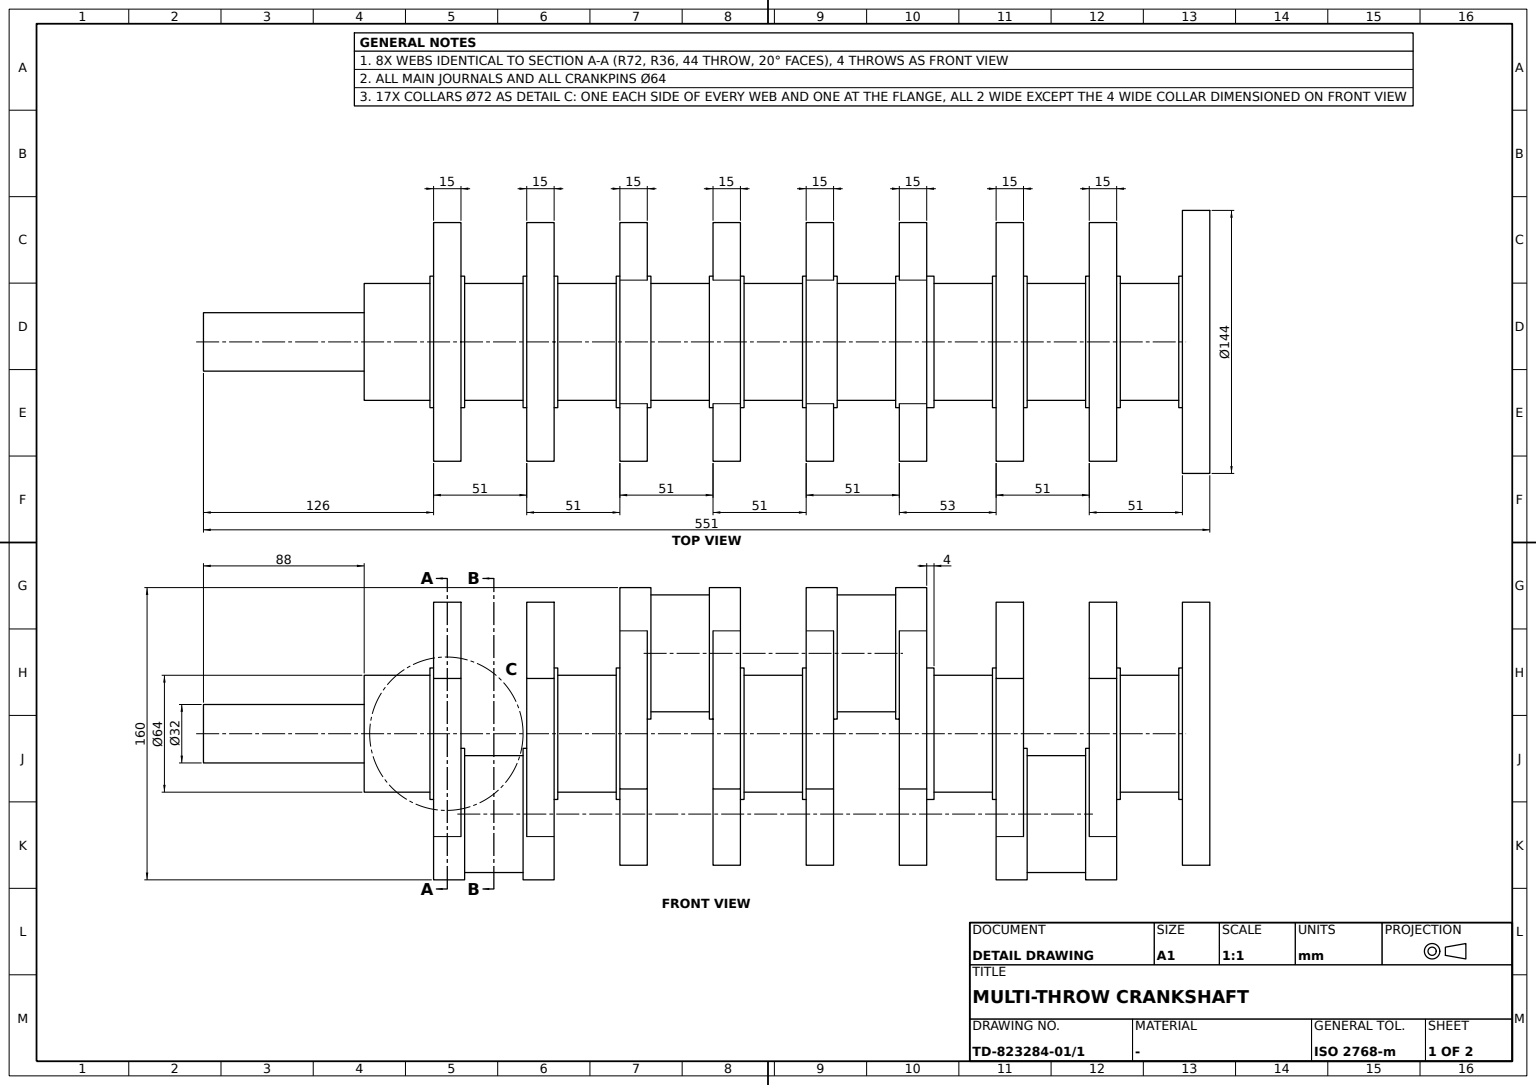
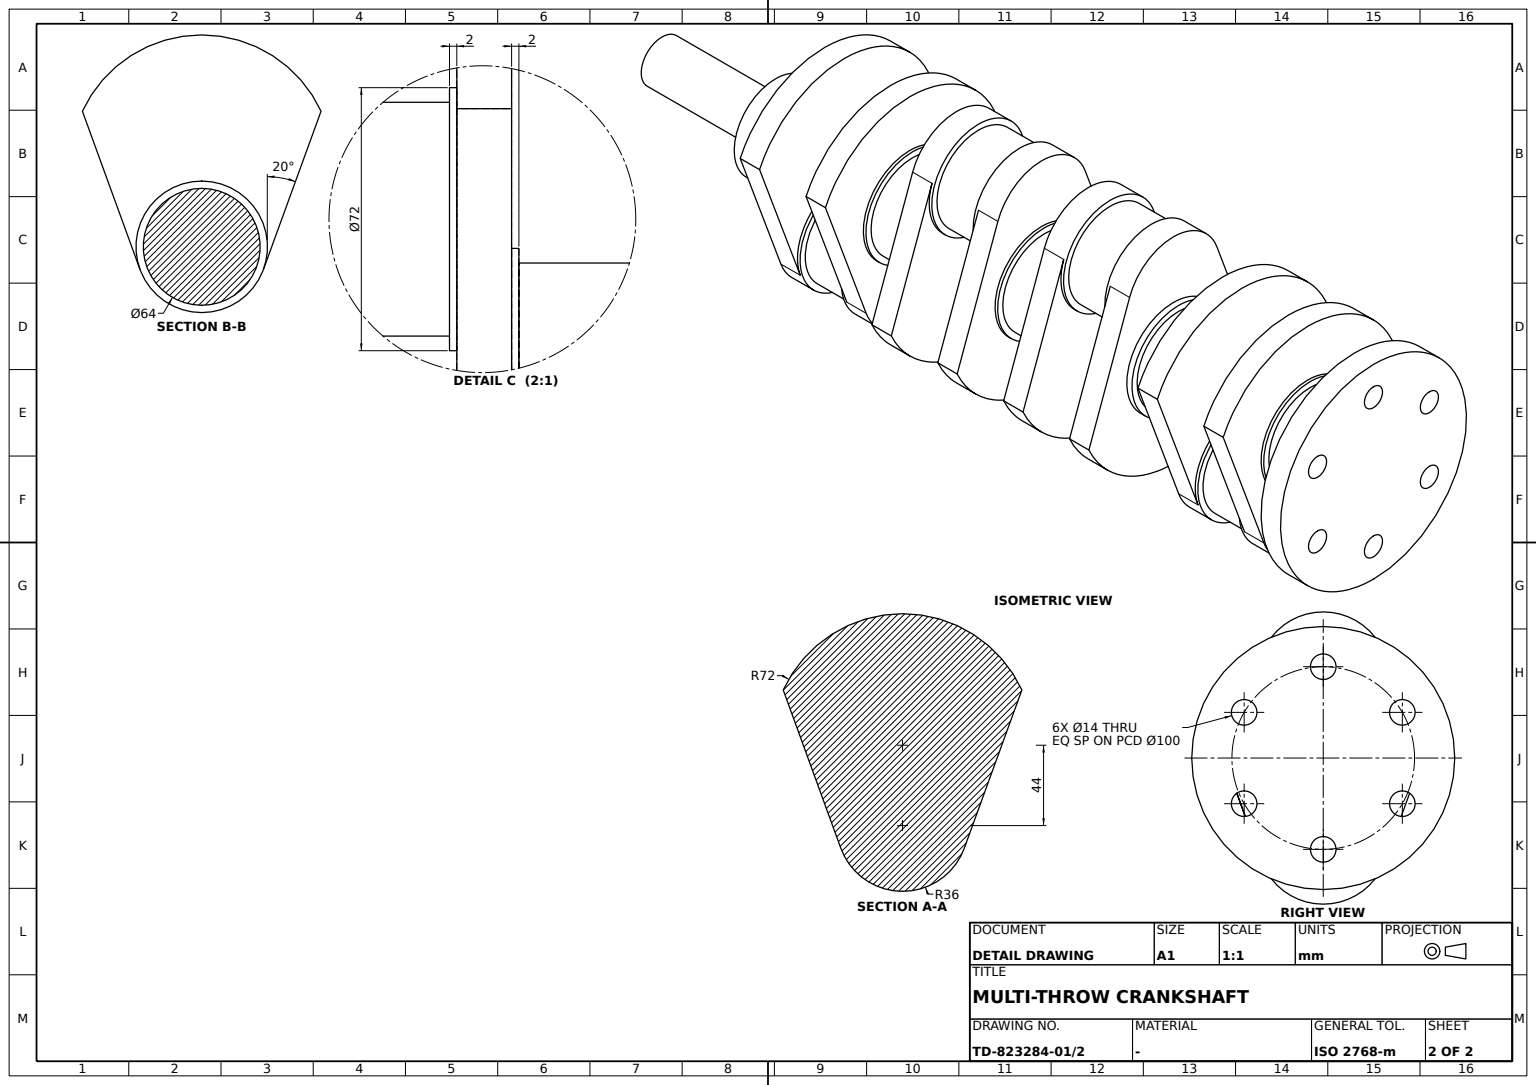
solid
v1 (502,0,-32)
v2 (502,0,32)
e1 v1 v2 CIRCLE(AX(P(502,0,0),D(1,0,0),D(0,1,0)),32)
e2 v2 v1 CIRCLE(AX(P(502,0,0),D(1,0,0),D(0,1,0)),32)
v3 (502,0,-36)
v4 (502,0,36)
e3 v3 v4 CIRCLE(AX(P(502,0,0),D(1,0,0),D(0,1,0)),36)
e4 v4 v3 CIRCLE(AX(P(502,0,0),D(1,0,0),D(0,1,0)),36)
face PLANE(AX(P(502,0,0),D(1,0,0),D(0,0,-1))) [-e1 -e2] [e3 e4]
v5 (296,0,-36)
v6 (296,0,36)
e5 v5 v6 CIRCLE(AX(P(296,0,0),D(1,0,0),D(0,1,0)),36)
v7 (294,0,-36)
e6 v7 v5 LINE
v8 (294,0,36)
e7 v7 v8 CIRCLE(AX(P(294,0,0),D(1,0,0),D(0,1,0)),36)
e8 v6 v8 LINE
face CYL(AX(P(296,0,0),D(-1,0,0),D(0,0,1)),36) [-e5 -e6 e7 -e8]
v9 (500,0,-36)
e9 v9 v3 LINE
v10 (500,0,36)
e10 v9 v10 CIRCLE(AX(P(500,0,0),D(1,0,0),D(0,1,0)),36)
e11 v4 v10 LINE
face CYL(AX(P(502,0,0),D(-1,0,0),D(0,0,1)),36) [-e3 -e9 e10 -e11]
v11 (143,0,-76)
v12 (143,0,-12)
e12 v11 v12 CIRCLE(AX(P(143,0,-44),D(1,0,0),D(0,1,0)),32)
v13 (175,0,-12)
e13 v13 v12 LINE
v14 (175,0,-76)
e14 v14 v13 CIRCLE(AX(P(175,0,-44),D(1,0,0),D(0,1,0)),32)
e15 v11 v14 LINE
face CYL(AX(P(175,0,-44),D(-1,0,0),D(0,0,1)),32) [e12 -e13 -e14 -e15]
v15 (449,65.336033,30.252318)
v16 (434,65.336033,30.252318)
e16 v15 v16 LINE
v17 (449,33.828934,-56.312725)
e17 v17 v15 LINE
v18 (434,33.828934,-56.312725)
e18 v17 v18 LINE
e19 v18 v16 LINE
face PLANE(AX(P(449,33.828934,-56.312725),D(0,-0.939692621,0.342020143),D(0,-0.342020143,-0.939692621))) rev [-e16 -e17 e18 e19]
v19 (396,65.336033,-30.252318)
v20 (396,33.828934,56.312725)
e20 v19 v20 LINE
v21 (381,65.336033,-30.252318)
e21 v19 v21 LINE
v22 (381,33.828934,56.312725)
e22 v21 v22 LINE
e23 v20 v22 LINE
face PLANE(AX(P(396,65.336033,-30.252318),D(0,-0.939692621,-0.342020143),D(0,0.342020143,-0.939692621))) rev [-e20 e21 e22 -e23]
v23 (449,0,72)
v24 (449,-65.336033,30.252318)
e24 v23 v24 CIRCLE(AX(P(449,0,0),D(1,0,0),D(0,0,-1)),72)
v25 (434,0,72)
e25 v23 v25 LINE
v26 (434,-65.336033,30.252318)
e26 v25 v26 CIRCLE(AX(P(434,0,0),D(1,0,0),D(0,0,-1)),72)
e27 v24 v26 LINE
face CYL(AX(P(449,0,0),D(-1,0,0),D(0,0,1)),72) [-e24 e25 e26 -e27]
v27 (294,65.336033,-30.252318)
v28 (294,33.828934,56.312725)
e28 v27 v28 LINE
v29 (294,0,80)
e29 v28 v29 CIRCLE(AX(P(294,0,44),D(1,0,0),D(0,0,-1)),36)
v30 (294,-33.828934,56.312725)
e30 v29 v30 CIRCLE(AX(P(294,0,44),D(1,0,0),D(0,0,-1)),36)
v31 (294,-65.336033,-30.252318)
e31 v30 v31 LINE
e32 v31 v27 CIRCLE(AX(P(294,0,0),D(1,0,0),D(0,0,-1)),72)
e33 v8 v7 CIRCLE(AX(P(294,0,0),D(1,0,0),D(0,1,0)),36)
face PLANE(AX(P(294,0,0),D(1,0,0),D(0,0,-1))) [e28 e29 e30 e31 e32] [-e7 -e33]
v32 (192,-33.828934,-56.312725)
v33 (192,0,-80)
e34 v32 v33 CIRCLE(AX(P(192,0,-44),D(1,0,0),D(0,0,-1)),36)
v34 (177,-33.828934,-56.312725)
e35 v32 v34 LINE
v35 (177,0,-8)
e36 v35 v34 CIRCLE(AX(P(177,0,-44),D(1,0,0),D(0,0,-1)),36)
v36 (175,0,-8)
e37 v35 v36 LINE
v37 (175,0,-80)
e38 v36 v37 CIRCLE(AX(P(175,0,-44),D(1,0,0),D(0,0,-1)),36)
e39 v37 v33 LINE
face CYL(AX(P(177,0,-44),D(-1,0,0),D(0,0,1)),36) [-e34 e35 -e36 e37 e38 e39]
v38 (279,-65.336033,-30.252318)
e40 v31 v38 LINE
v39 (279,-33.828934,56.312725)
e41 v30 v39 LINE
e42 v39 v38 LINE
face PLANE(AX(P(294,-33.828934,56.312725),D(0,0.939692621,-0.342020143),D(0,0.342020143,0.939692621))) rev [-e40 -e31 e41 e42]
v40 (243,0,8)
v41 (245,0,8)
e43 v40 v41 LINE
v42 (245,0,80)
e44 v42 v41 CIRCLE(AX(P(245,0,44),D(1,0,0),D(0,1,0)),36)
v43 (228,0,80)
e45 v42 v43 LINE
v44 (228,-33.828934,56.312725)
e46 v43 v44 CIRCLE(AX(P(228,0,44),D(1,0,0),D(0,1,0)),36)
v45 (243,-33.828934,56.312725)
e47 v45 v44 LINE
e48 v40 v45 CIRCLE(AX(P(243,0,44),D(-1,0,0),D(0,1,0)),36)
face CYL(AX(P(243,0,44),D(-1,0,0),D(0,0,1)),36) [e43 -e44 e45 e46 -e47 -e48]
e49 v37 v36 CIRCLE(AX(P(175,0,-44),D(1,0,0),D(0,0,-1)),36)
v46 (177,33.828934,-56.312725)
e50 v46 v35 CIRCLE(AX(P(177,0,-44),D(1,0,0),D(0,0,-1)),36)
v47 (192,33.828934,-56.312725)
e51 v47 v46 LINE
e52 v33 v47 CIRCLE(AX(P(192,0,-44),D(1,0,0),D(0,0,-1)),36)
face CYL(AX(P(177,0,-44),D(-1,0,0),D(0,0,1)),36) [-e39 e49 -e37 -e50 -e51 -e52]
v48 (141,-33.828934,-56.312725)
v49 (141,0,-8)
e53 v48 v49 CIRCLE(AX(P(141,0,-44),D(-1,0,0),D(0,1,0)),36)
v50 (126,-33.828934,-56.312725)
e54 v48 v50 LINE
v51 (126,0,-80)
e55 v50 v51 CIRCLE(AX(P(126,0,-44),D(1,0,0),D(0,1,0)),36)
v52 (143,0,-80)
e56 v51 v52 LINE
v53 (143,0,-8)
e57 v53 v52 CIRCLE(AX(P(143,0,-44),D(1,0,0),D(0,1,0)),36)
e58 v53 v49 LINE
face CYL(AX(P(141,0,-44),D(-1,0,0),D(0,0,1)),36) [-e53 e54 e55 e56 -e57 e58]
v54 (551,0,72)
v55 (551,0,-72)
e59 v54 v55 CIRCLE(AX(P(551,0,0),D(1,0,0),D(0,1,0)),72)
e60 v55 v54 CIRCLE(AX(P(551,0,0),D(1,0,0),D(0,1,0)),72)
v56 (551,0,43)
v57 (551,0,57)
e61 v56 v57 CIRCLE(AX(P(551,0,50),D(1,0,0),D(0,1,0)),7)
e62 v57 v56 CIRCLE(AX(P(551,0,50),D(1,0,0),D(0,1,0)),7)
v58 (551,0,-57)
v59 (551,0,-43)
e63 v58 v59 CIRCLE(AX(P(551,0,-50),D(1,0,0),D(0,-1,0)),7)
e64 v59 v58 CIRCLE(AX(P(551,0,-50),D(1,0,0),D(0,-1,0)),7)
v60 (551,43.30127,32)
v61 (551,43.30127,18)
e65 v60 v61 CIRCLE(AX(P(551,43.30127,25),D(1,0,0),D(0,0.5,-0.866025404)),7)
e66 v61 v60 CIRCLE(AX(P(551,43.30127,25),D(1,0,0),D(0,0.5,-0.866025404)),7)
v62 (551,-43.30127,-18)
v63 (551,-43.30127,-32)
e67 v62 v63 CIRCLE(AX(P(551,-43.30127,-25),D(1,0,0),D(0,-0.5,0.866025404)),7)
e68 v63 v62 CIRCLE(AX(P(551,-43.30127,-25),D(1,0,0),D(0,-0.5,0.866025404)),7)
v64 (551,43.30127,-32)
v65 (551,43.30127,-18)
e69 v64 v65 CIRCLE(AX(P(551,43.30127,-25),D(1,0,0),D(0,-0.5,-0.866025404)),7)
e70 v65 v64 CIRCLE(AX(P(551,43.30127,-25),D(1,0,0),D(0,-0.5,-0.866025404)),7)
v66 (551,-43.30127,18)
v67 (551,-43.30127,32)
e71 v66 v67 CIRCLE(AX(P(551,-43.30127,25),D(1,0,0),D(0,0.5,0.866025404)),7)
e72 v67 v66 CIRCLE(AX(P(551,-43.30127,25),D(1,0,0),D(0,0.5,0.866025404)),7)
face PLANE(AX(P(551,0,0),D(1,0,0),D(0,0,-1))) [e59 e60] [-e61 -e62] [-e63 -e64] [-e65 -e66] [-e67 -e68] [-e69 -e70] [-e71 -e72]
e73 v13 v14 CIRCLE(AX(P(175,0,-44),D(1,0,0),D(0,1,0)),32)
face PLANE(AX(P(175,0,-44),D(1,0,0),D(0,0,-1))) rev [e14 e73] [-e49 -e38]
v68 (296,0,32)
v69 (328,0,32)
e74 v68 v69 LINE
v70 (328,0,-32)
e75 v70 v69 CIRCLE(AX(P(328,0,0),D(1,0,0),D(0,1,0)),32)
v71 (296,0,-32)
e76 v70 v71 LINE
e77 v71 v68 CIRCLE(AX(P(296,0,0),D(1,0,0),D(0,1,0)),32)
face CYL(AX(P(328,0,0),D(-1,0,0),D(0,0,1)),32) [e74 -e75 e76 e77]
v72 (379,0,8)
v73 (379,0,80)
e78 v72 v73 CIRCLE(AX(P(379,0,44),D(1,0,0),D(0,1,0)),36)
e79 v73 v72 CIRCLE(AX(P(379,0,44),D(1,0,0),D(0,1,0)),36)
v74 (379,0,76)
v75 (379,0,12)
e80 v74 v75 CIRCLE(AX(P(379,0,44),D(1,0,0),D(0,1,0)),32)
e81 v75 v74 CIRCLE(AX(P(379,0,44),D(1,0,0),D(0,1,0)),32)
face PLANE(AX(P(379,0,44),D(1,0,0),D(0,0,-1))) rev [-e78 -e79] [e80 e81]
v76 (141,33.828934,-56.312725)
v77 (141,65.336033,30.252318)
e82 v76 v77 LINE
v78 (126,33.828934,-56.312725)
e83 v76 v78 LINE
v79 (126,65.336033,30.252318)
e84 v78 v79 LINE
e85 v77 v79 LINE
face PLANE(AX(P(141,33.828934,-56.312725),D(0,-0.939692621,0.342020143),D(0,-0.342020143,-0.939692621))) rev [-e82 e83 e84 -e85]
e86 v41 v42 CIRCLE(AX(P(245,0,44),D(1,0,0),D(0,1,0)),36)
v80 (245,0,76)
v81 (245,0,12)
e87 v80 v81 CIRCLE(AX(P(245,0,44),D(1,0,0),D(0,1,0)),32)
e88 v81 v80 CIRCLE(AX(P(245,0,44),D(1,0,0),D(0,1,0)),32)
face PLANE(AX(P(245,0,44),D(1,0,0),D(0,0,-1))) [e86 e44] [-e87 -e88]
v82 (277,0,8)
v83 (279,0,8)
e89 v82 v83 LINE
v84 (277,0,80)
e90 v82 v84 CIRCLE(AX(P(277,0,44),D(1,0,0),D(0,1,0)),36)
e91 v29 v84 LINE
v85 (279,33.828934,56.312725)
e92 v28 v85 LINE
e93 v83 v85 CIRCLE(AX(P(279,0,44),D(1,0,0),D(0,1,0)),36)
face CYL(AX(P(279,0,44),D(-1,0,0),D(0,0,1)),36) [-e89 e90 -e91 -e29 e92 -e93]
v86 (228,-65.336033,-30.252318)
e94 v44 v86 LINE
v87 (243,-65.336033,-30.252318)
e95 v87 v86 LINE
e96 v45 v87 LINE
face PLANE(AX(P(243,-33.828934,56.312725),D(0,0.939692621,-0.342020143),D(0,0.342020143,0.939692621))) rev [e94 -e95 -e96 e47]
v88 (277,0,76)
e97 v80 v88 LINE
v89 (277,0,12)
e98 v89 v88 CIRCLE(AX(P(277,0,44),D(1,0,0),D(0,1,0)),32)
e99 v89 v81 LINE
face CYL(AX(P(277,0,44),D(-1,0,0),D(0,0,1)),32) [e88 e97 -e98 e99]
v90 (347,0,8)
v91 (347,0,80)
e100 v90 v91 CIRCLE(AX(P(347,0,44),D(1,0,0),D(0,1,0)),36)
e101 v91 v90 CIRCLE(AX(P(347,0,44),D(1,0,0),D(0,1,0)),36)
v92 (347,0,76)
v93 (347,0,12)
e102 v92 v93 CIRCLE(AX(P(347,0,44),D(1,0,0),D(0,1,0)),32)
e103 v93 v92 CIRCLE(AX(P(347,0,44),D(1,0,0),D(0,1,0)),32)
face PLANE(AX(P(347,0,44),D(1,0,0),D(0,0,-1))) [e100 e101] [-e102 -e103]
v94 (536,-43.30127,-32)
v95 (536,-43.30127,-18)
e104 v94 v95 CIRCLE(AX(P(536,-43.30127,-25),D(1,0,0),D(0,-0.5,0.866025404)),7)
e105 v94 v63 LINE
e106 v62 v95 LINE
face CYL(AX(P(536,-43.30127,-25),D(1,0,0),D(0,0,-1)),7) rev [-e104 e105 e68 e106]
v96 (432,0,36)
v97 (432,0,-36)
e107 v96 v97 CIRCLE(AX(P(432,0,0),D(1,0,0),D(0,1,0)),36)
e108 v97 v96 CIRCLE(AX(P(432,0,0),D(1,0,0),D(0,1,0)),36)
v98 (432,0,-32)
v99 (432,0,32)
e109 v98 v99 CIRCLE(AX(P(432,0,0),D(1,0,0),D(0,1,0)),32)
e110 v99 v98 CIRCLE(AX(P(432,0,0),D(1,0,0),D(0,1,0)),32)
face PLANE(AX(P(432,0,0),D(1,0,0),D(0,0,-1))) rev [-e107 -e108] [e109 e110]
v100 (328,0,-36)
v101 (330,0,-36)
e111 v100 v101 LINE
v102 (328,0,36)
e112 v100 v102 CIRCLE(AX(P(328,0,0),D(1,0,0),D(0,1,0)),36)
v103 (330,0,36)
e113 v103 v102 LINE
e114 v101 v103 CIRCLE(AX(P(330,0,0),D(1,0,0),D(0,1,0)),36)
face CYL(AX(P(330,0,0),D(-1,0,0),D(0,0,1)),36) [-e111 e112 -e113 -e114]
v104 (194,0,36)
v105 (194,0,-36)
e115 v104 v105 CIRCLE(AX(P(194,0,0),D(1,0,0),D(0,0,-1)),36)
v106 (192,0,36)
e116 v104 v106 LINE
v107 (192,0,-36)
e117 v106 v107 CIRCLE(AX(P(192,0,0),D(1,0,0),D(0,0,-1)),36)
e118 v107 v105 LINE
face CYL(AX(P(194,0,0),D(-1,0,0),D(0,0,1)),36) [-e115 e116 e117 e118]
v108 (536,0,43)
v109 (536,0,57)
e119 v108 v109 CIRCLE(AX(P(536,0,50),D(1,0,0),D(0,1,0)),7)
e120 v109 v108 CIRCLE(AX(P(536,0,50),D(1,0,0),D(0,1,0)),7)
v110 (536,0,72)
v111 (536,0,-72)
e121 v110 v111 CIRCLE(AX(P(536,0,0),D(1,0,0),D(0,1,0)),72)
e122 v111 v110 CIRCLE(AX(P(536,0,0),D(1,0,0),D(0,1,0)),72)
e123 v95 v94 CIRCLE(AX(P(536,-43.30127,-25),D(1,0,0),D(0,-0.5,0.866025404)),7)
v112 (536,43.30127,18)
v113 (536,43.30127,32)
e124 v112 v113 CIRCLE(AX(P(536,43.30127,25),D(1,0,0),D(0,0.5,-0.866025404)),7)
e125 v113 v112 CIRCLE(AX(P(536,43.30127,25),D(1,0,0),D(0,0.5,-0.866025404)),7)
v114 (536,0,-43)
v115 (536,0,-57)
e126 v114 v115 CIRCLE(AX(P(536,0,-50),D(1,0,0),D(0,-1,0)),7)
e127 v115 v114 CIRCLE(AX(P(536,0,-50),D(1,0,0),D(0,-1,0)),7)
v116 (536,0,36)
v117 (536,0,-36)
e128 v116 v117 CIRCLE(AX(P(536,0,0),D(1,0,0),D(0,1,0)),36)
e129 v117 v116 CIRCLE(AX(P(536,0,0),D(1,0,0),D(0,1,0)),36)
v118 (536,-43.30127,18)
v119 (536,-43.30127,32)
e130 v118 v119 CIRCLE(AX(P(536,-43.30127,25),D(1,0,0),D(0,0.5,0.866025404)),7)
e131 v119 v118 CIRCLE(AX(P(536,-43.30127,25),D(1,0,0),D(0,0.5,0.866025404)),7)
v120 (536,43.30127,-18)
v121 (536,43.30127,-32)
e132 v120 v121 CIRCLE(AX(P(536,43.30127,-25),D(1,0,0),D(0,-0.5,-0.866025404)),7)
e133 v121 v120 CIRCLE(AX(P(536,43.30127,-25),D(1,0,0),D(0,-0.5,-0.866025404)),7)
face PLANE(AX(P(536,0,0),D(1,0,0),D(0,0,-1))) rev [e119 e120] [-e121 -e122] [e123 e104] [e124 e125] [e126 e127] [e128 e129] [e130 e131] [e132 e133]
v122 (451,0,-76)
v123 (451,0,-12)
e134 v122 v123 CIRCLE(AX(P(451,0,-44),D(1,0,0),D(0,1,0)),32)
e135 v123 v122 CIRCLE(AX(P(451,0,-44),D(1,0,0),D(0,1,0)),32)
v124 (451,0,-8)
v125 (451,0,-80)
e136 v124 v125 CIRCLE(AX(P(451,0,-44),D(1,0,0),D(0,1,0)),36)
e137 v125 v124 CIRCLE(AX(P(451,0,-44),D(1,0,0),D(0,1,0)),36)
face PLANE(AX(P(451,0,-44),D(1,0,0),D(0,0,-1))) [-e134 -e135] [e136 e137]
v126 (330,0,80)
e138 v126 v91 LINE
v127 (330,-33.828934,56.312725)
e139 v126 v127 CIRCLE(AX(P(330,0,44),D(1,0,0),D(0,0,-1)),36)
v128 (345,-33.828934,56.312725)
e140 v128 v127 LINE
v129 (345,0,8)
e141 v129 v128 CIRCLE(AX(P(345,0,44),D(-1,0,0),D(0,1,0)),36)
e142 v90 v129 LINE
face CYL(AX(P(345,0,44),D(-1,0,0),D(0,0,1)),36) [-e138 e139 -e140 -e141 -e142 -e101]
v130 (124,0,32)
v131 (88,0,32)
e143 v130 v131 LINE
v132 (88,0,-32)
e144 v131 v132 CIRCLE(AX(P(88,0,0),D(1,0,0),D(0,1,0)),32)
v133 (124,0,-32)
e145 v132 v133 LINE
e146 v130 v133 CIRCLE(AX(P(124,0,0),D(1,0,0),D(0,1,0)),32)
face CYL(AX(P(124,0,0),D(-1,0,0),D(0,0,1)),32) [e143 e144 e145 -e146]
v134 (228,33.828934,56.312725)
e147 v134 v43 CIRCLE(AX(P(228,0,44),D(1,0,0),D(0,1,0)),36)
v135 (228,65.336033,-30.252318)
e148 v135 v134 LINE
e149 v86 v135 CIRCLE(AX(P(228,0,0),D(1,0,0),D(0,1,0)),72)
v136 (228,0,36)
v137 (228,0,-36)
e150 v136 v137 CIRCLE(AX(P(228,0,0),D(1,0,0),D(0,0,-1)),36)
e151 v137 v136 CIRCLE(AX(P(228,0,0),D(1,0,0),D(0,0,-1)),36)
face PLANE(AX(P(228,0,0),D(1,0,0),D(0,0,-1))) rev [-e94 -e46 -e147 -e148 -e149] [e150 e151]
v138 (226,0,36)
e152 v136 v138 LINE
v139 (226,0,-36)
e153 v139 v137 LINE
e154 v139 v138 CIRCLE(AX(P(226,0,0),D(1,0,0),D(0,0,-1)),36)
face CYL(AX(P(228,0,0),D(-1,0,0),D(0,0,1)),36) [-e152 -e151 -e153 e154]
v140 (279,65.336033,-30.252318)
e155 v140 v85 LINE
e156 v38 v140 CIRCLE(AX(P(279,0,0),D(1,0,0),D(0,0,-1)),72)
e157 v39 v83 CIRCLE(AX(P(279,0,44),D(1,0,0),D(0,1,0)),36)
face PLANE(AX(P(279,0,0),D(1,0,0),D(0,0,-1))) rev [-e155 -e156 -e42 e157 e93]
v141 (396,-65.336033,-30.252318)
e158 v141 v19 CIRCLE(AX(P(396,0,0),D(1,0,0),D(0,0,-1)),72)
v142 (381,-65.336033,-30.252318)
e159 v141 v142 LINE
e160 v142 v21 CIRCLE(AX(P(381,0,0),D(1,0,0),D(0,0,-1)),72)
face CYL(AX(P(396,0,0),D(-1,0,0),D(0,0,1)),72) [-e21 -e158 e159 e160]
e161 v133 v130 CIRCLE(AX(P(124,0,0),D(1,0,0),D(0,1,0)),32)
e162 v132 v131 CIRCLE(AX(P(88,0,0),D(1,0,0),D(0,1,0)),32)
face CYL(AX(P(124,0,0),D(-1,0,0),D(0,0,1)),32) [-e143 -e161 -e145 e162]
v143 (192,65.336033,30.252318)
v144 (192,0,72)
e163 v143 v144 CIRCLE(AX(P(192,0,0),D(1,0,0),D(0,0,-1)),72)
v145 (177,65.336033,30.252318)
e164 v143 v145 LINE
v146 (177,0,72)
e165 v145 v146 CIRCLE(AX(P(177,0,0),D(1,0,0),D(0,0,-1)),72)
e166 v144 v146 LINE
face CYL(AX(P(192,0,0),D(-1,0,0),D(0,0,1)),72) [-e163 e164 e165 -e166]
v147 (483,0,-76)
v148 (483,0,-12)
e167 v147 v148 CIRCLE(AX(P(483,0,-44),D(1,0,0),D(0,1,0)),32)
e168 v147 v122 LINE
e169 v123 v148 LINE
face CYL(AX(P(483,0,-44),D(-1,0,0),D(0,0,1)),32) [-e167 e168 e134 e169]
e170 v110 v54 LINE
e171 v55 v111 LINE
face CYL(AX(P(551,0,0),D(-1,0,0),D(0,0,1)),72) [e122 e170 -e60 e171]
v149 (500,65.336033,30.252318)
v150 (500,0,72)
e172 v149 v150 CIRCLE(AX(P(500,0,0),D(1,0,0),D(0,0,-1)),72)
v151 (485,65.336033,30.252318)
e173 v149 v151 LINE
v152 (485,0,72)
e174 v151 v152 CIRCLE(AX(P(485,0,0),D(1,0,0),D(0,0,-1)),72)
e175 v150 v152 LINE
face CYL(AX(P(500,0,0),D(-1,0,0),D(0,0,1)),72) [-e172 e173 e174 -e175]
e176 v16 v25 CIRCLE(AX(P(434,0,0),D(1,0,0),D(0,0,-1)),72)
e177 v15 v23 CIRCLE(AX(P(449,0,0),D(1,0,0),D(0,0,-1)),72)
face CYL(AX(P(449,0,0),D(-1,0,0),D(0,0,1)),72) [e176 -e25 -e177 e16]
v153 (485,33.828934,-56.312725)
v154 (485,0,-8)
e178 v153 v154 CIRCLE(AX(P(485,0,-44),D(1,0,0),D(0,1,0)),36)
v155 (485,-33.828934,-56.312725)
e179 v154 v155 CIRCLE(AX(P(485,0,-44),D(1,0,0),D(0,1,0)),36)
v156 (485,-65.336033,30.252318)
e180 v156 v155 LINE
e181 v152 v156 CIRCLE(AX(P(485,0,0),D(1,0,0),D(0,0,-1)),72)
e182 v153 v151 LINE
face PLANE(AX(P(485,0,-44),D(1,0,0),D(0,0,-1))) rev [e178 e179 -e180 -e181 -e174 -e182]
e183 v108 v56 LINE
e184 v57 v109 LINE
face CYL(AX(P(536,0,50),D(1,0,0),D(0,0,-1)),7) rev [e62 -e183 -e120 -e184]
v157 (0,0,16)
v158 (0,0,-16)
e185 v157 v158 CIRCLE(AX(P(0,0,0),D(1,0,0),D(0,1,0)),16)
e186 v158 v157 CIRCLE(AX(P(0,0,0),D(1,0,0),D(0,1,0)),16)
face PLANE(AX(P(0,0,0),D(1,0,0),D(0,0,-1))) rev [-e185 -e186]
e187 v51 v78 CIRCLE(AX(P(126,0,-44),D(1,0,0),D(0,1,0)),36)
v159 (126,-65.336033,30.252318)
e188 v159 v50 LINE
v160 (126,0,72)
e189 v160 v159 CIRCLE(AX(P(126,0,0),D(1,0,0),D(0,1,0)),72)
e190 v79 v160 CIRCLE(AX(P(126,0,0),D(1,0,0),D(0,1,0)),72)
v161 (126,0,36)
v162 (126,0,-36)
e191 v161 v162 CIRCLE(AX(P(126,0,0),D(1,0,0),D(0,1,0)),36)
e192 v162 v161 CIRCLE(AX(P(126,0,0),D(1,0,0),D(0,1,0)),36)
face PLANE(AX(P(126,0,-44),D(1,0,0),D(0,0,-1))) rev [-e84 -e187 -e55 -e188 -e189 -e190] [e191 e192]
e193 v88 v89 CIRCLE(AX(P(277,0,44),D(1,0,0),D(0,1,0)),32)
e194 v84 v82 CIRCLE(AX(P(277,0,44),D(1,0,0),D(0,1,0)),36)
face PLANE(AX(P(277,0,44),D(1,0,0),D(0,0,-1))) rev [e193 e98] [-e90 -e194]
e195 v119 v67 LINE
e196 v66 v118 LINE
face CYL(AX(P(536,-43.30127,25),D(1,0,0),D(0,0,-1)),7) rev [-e195 -e130 -e196 e71]
v163 (194,0,32)
v164 (194,0,-32)
e197 v163 v164 CIRCLE(AX(P(194,0,0),D(1,0,0),D(0,0,-1)),32)
e198 v164 v163 CIRCLE(AX(P(194,0,0),D(1,0,0),D(0,0,-1)),32)
e199 v105 v104 CIRCLE(AX(P(194,0,0),D(1,0,0),D(0,0,-1)),36)
face PLANE(AX(P(194,0,0),D(1,0,0),D(0,0,-1))) [-e197 -e198] [e199 e115]
e200 v112 v61 LINE
e201 v60 v113 LINE
face CYL(AX(P(536,43.30127,25),D(1,0,0),D(0,0,-1)),7) rev [e65 -e200 -e125 -e201]
v165 (124,0,36)
e202 v161 v165 LINE
v166 (124,0,-36)
e203 v165 v166 CIRCLE(AX(P(124,0,0),D(1,0,0),D(0,1,0)),36)
e204 v166 v162 LINE
face CYL(AX(P(126,0,0),D(-1,0,0),D(0,0,1)),36) [-e191 e202 e203 e204]
v167 (88,0,-16)
e205 v158 v167 LINE
v168 (88,0,16)
e206 v168 v167 CIRCLE(AX(P(88,0,0),D(1,0,0),D(0,1,0)),16)
e207 v168 v157 LINE
face CYL(AX(P(88,0,0),D(-1,0,0),D(0,0,1)),16) [e185 e205 -e206 e207]
v169 (434,-33.828934,-56.312725)
v170 (434,0,-80)
e208 v169 v170 CIRCLE(AX(P(434,0,-44),D(1,0,0),D(0,0,-1)),36)
e209 v26 v169 LINE
e210 v170 v18 CIRCLE(AX(P(434,0,-44),D(1,0,0),D(0,0,-1)),36)
v171 (434,0,36)
v172 (434,0,-36)
e211 v171 v172 CIRCLE(AX(P(434,0,0),D(1,0,0),D(0,1,0)),36)
e212 v172 v171 CIRCLE(AX(P(434,0,0),D(1,0,0),D(0,1,0)),36)
face PLANE(AX(P(434,0,-44),D(1,0,0),D(0,0,-1))) rev [-e208 -e209 -e26 -e176 -e19 -e210] [e211 e212]
e213 v59 v114 LINE
e214 v115 v58 LINE
face CYL(AX(P(536,0,-50),D(1,0,0),D(0,0,-1)),7) rev [-e213 e64 -e214 -e126]
v173 (141,-65.336033,30.252318)
e215 v173 v159 LINE
v174 (141,0,72)
e216 v174 v173 CIRCLE(AX(P(141,0,0),D(1,0,0),D(0,1,0)),72)
e217 v174 v160 LINE
face CYL(AX(P(141,0,0),D(-1,0,0),D(0,0,1)),72) [e189 -e215 -e216 e217]
v175 (396,0,-36)
v176 (396,0,36)
e218 v175 v176 CIRCLE(AX(P(396,0,0),D(1,0,0),D(0,1,0)),36)
e219 v176 v175 CIRCLE(AX(P(396,0,0),D(1,0,0),D(0,1,0)),36)
v177 (396,0,80)
e220 v20 v177 CIRCLE(AX(P(396,0,44),D(1,0,0),D(0,0,-1)),36)
v178 (396,-33.828934,56.312725)
e221 v177 v178 CIRCLE(AX(P(396,0,44),D(1,0,0),D(0,0,-1)),36)
e222 v178 v141 LINE
face PLANE(AX(P(396,0,0),D(1,0,0),D(0,0,-1))) [-e218 -e219] [e20 e220 e221 e222 e158]
e223 v12 v11 CIRCLE(AX(P(143,0,-44),D(1,0,0),D(0,1,0)),32)
face CYL(AX(P(175,0,-44),D(-1,0,0),D(0,0,1)),32) [e223 e15 -e73 e13]
e224 v102 v100 CIRCLE(AX(P(328,0,0),D(1,0,0),D(0,1,0)),36)
e225 v69 v70 CIRCLE(AX(P(328,0,0),D(1,0,0),D(0,1,0)),32)
face PLANE(AX(P(328,0,0),D(1,0,0),D(0,0,-1))) rev [-e112 -e224] [e225 e75]
v179 (345,65.336033,-30.252318)
v180 (345,33.828934,56.312725)
e226 v179 v180 LINE
e227 v180 v129 CIRCLE(AX(P(345,0,44),D(-1,0,0),D(0,1,0)),36)
v181 (345,-65.336033,-30.252318)
e228 v128 v181 LINE
e229 v181 v179 CIRCLE(AX(P(345,0,0),D(1,0,0),D(0,0,-1)),72)
face PLANE(AX(P(345,0,0),D(1,0,0),D(0,0,-1))) [e226 e227 e141 e228 e229]
v182 (534,0,32)
e230 v2 v182 LINE
v183 (534,0,-32)
e231 v183 v182 CIRCLE(AX(P(534,0,0),D(1,0,0),D(0,1,0)),32)
e232 v183 v1 LINE
face CYL(AX(P(534,0,0),D(-1,0,0),D(0,0,1)),32) [e1 e230 -e231 e232]
face CYL(AX(P(536,43.30127,25),D(1,0,0),D(0,0,-1)),7) rev [e201 -e124 e200 e66]
e233 v10 v9 CIRCLE(AX(P(500,0,0),D(1,0,0),D(0,1,0)),36)
face CYL(AX(P(502,0,0),D(-1,0,0),D(0,0,1)),36) [e9 -e4 e11 e233]
face CYL(AX(P(536,-43.30127,25),D(1,0,0),D(0,0,-1)),7) rev [e72 e196 -e131 e195]
e234 v167 v168 CIRCLE(AX(P(88,0,0),D(1,0,0),D(0,1,0)),16)
face PLANE(AX(P(88,0,0),D(1,0,0),D(0,0,-1))) rev [-e162 -e144] [e206 e234]
e235 v49 v76 CIRCLE(AX(P(141,0,-44),D(-1,0,0),D(0,1,0)),36)
e236 v52 v53 CIRCLE(AX(P(143,0,-44),D(1,0,0),D(0,1,0)),36)
face CYL(AX(P(141,0,-44),D(-1,0,0),D(0,0,1)),36) [-e235 -e58 -e236 -e56 e187 -e83]
v184 (534,0,-36)
v185 (534,0,36)
e237 v184 v185 CIRCLE(AX(P(534,0,0),D(1,0,0),D(0,1,0)),36)
e238 v116 v185 LINE
e239 v184 v117 LINE
face CYL(AX(P(536,0,0),D(-1,0,0),D(0,0,1)),36) [e237 -e238 -e129 -e239]
e240 v166 v165 CIRCLE(AX(P(124,0,0),D(1,0,0),D(0,1,0)),36)
face CYL(AX(P(126,0,0),D(-1,0,0),D(0,0,1)),36) [-e202 -e192 -e204 e240]
face CYL(AX(P(279,0,44),D(-1,0,0),D(0,0,1)),36) [-e41 -e30 e91 e194 e89 -e157]
v186 (243,33.828934,56.312725)
e241 v186 v40 CIRCLE(AX(P(243,0,44),D(-1,0,0),D(0,1,0)),36)
e242 v186 v134 LINE
face CYL(AX(P(243,0,44),D(-1,0,0),D(0,0,1)),36) [-e45 -e86 -e43 -e241 e242 e147]
e243 v120 v65 LINE
e244 v64 v121 LINE
face CYL(AX(P(536,43.30127,-25),D(1,0,0),D(0,0,-1)),7) rev [-e132 e243 e70 e244]
e245 v182 v183 CIRCLE(AX(P(534,0,0),D(1,0,0),D(0,1,0)),32)
face CYL(AX(P(534,0,0),D(-1,0,0),D(0,0,1)),32) [-e245 -e230 e2 -e232]
face PLANE(AX(P(143,0,-44),D(1,0,0),D(0,0,-1))) [e236 e57] [-e12 -e223]
v187 (226,0,-32)
v188 (226,0,32)
e246 v187 v188 CIRCLE(AX(P(226,0,0),D(1,0,0),D(0,0,-1)),32)
e247 v187 v164 LINE
e248 v163 v188 LINE
face CYL(AX(P(226,0,0),D(-1,0,0),D(0,0,1)),32) [-e246 e247 e198 e248]
e249 v6 v5 CIRCLE(AX(P(296,0,0),D(1,0,0),D(0,1,0)),36)
e250 v68 v71 CIRCLE(AX(P(296,0,0),D(1,0,0),D(0,1,0)),32)
face PLANE(AX(P(296,0,0),D(1,0,0),D(0,0,-1))) [e249 e5] [-e77 -e250]
v189 (500,-33.828934,-56.312725)
v190 (500,0,-80)
e251 v189 v190 CIRCLE(AX(P(500,0,-44),D(1,0,0),D(0,0,-1)),36)
v191 (500,33.828934,-56.312725)
e252 v190 v191 CIRCLE(AX(P(500,0,-44),D(1,0,0),D(0,0,-1)),36)
e253 v191 v149 LINE
v192 (500,-65.336033,30.252318)
e254 v150 v192 CIRCLE(AX(P(500,0,0),D(1,0,0),D(0,0,-1)),72)
e255 v192 v189 LINE
face PLANE(AX(P(500,0,-44),D(1,0,0),D(0,0,-1))) [-e233 -e10] [e251 e252 e253 e172 e254 e255]
face CYL(AX(P(296,0,0),D(-1,0,0),D(0,0,1)),36) [-e249 e8 e33 e6]
e256 v148 v147 CIRCLE(AX(P(483,0,-44),D(1,0,0),D(0,1,0)),32)
face CYL(AX(P(483,0,-44),D(-1,0,0),D(0,0,1)),32) [-e168 -e256 -e169 e135]
e257 v92 v74 LINE
e258 v75 v93 LINE
face CYL(AX(P(379,0,44),D(-1,0,0),D(0,0,1)),32) [e103 e257 -e81 e258]
v193 (400,0,36)
v194 (400,0,-36)
e259 v193 v194 CIRCLE(AX(P(400,0,0),D(1,0,0),D(0,1,0)),36)
e260 v194 v193 CIRCLE(AX(P(400,0,0),D(1,0,0),D(0,1,0)),36)
v195 (400,0,-32)
v196 (400,0,32)
e261 v195 v196 CIRCLE(AX(P(400,0,0),D(1,0,0),D(0,1,0)),32)
e262 v196 v195 CIRCLE(AX(P(400,0,0),D(1,0,0),D(0,1,0)),32)
face PLANE(AX(P(400,0,0),D(1,0,0),D(0,0,-1))) [e259 e260] [-e261 -e262]
e263 v27 v140 LINE
face PLANE(AX(P(294,65.336033,-30.252318),D(0,-0.939692621,-0.342020143),D(0,0.342020143,-0.939692621))) rev [-e92 -e28 e263 e155]
e264 v193 v176 LINE
e265 v175 v194 LINE
face CYL(AX(P(398,0,0),D(-1,0,0),D(0,0,1)),36) [-e259 e264 e219 e265]
v197 (243,65.336033,-30.252318)
e266 v197 v135 LINE
e267 v87 v197 CIRCLE(AX(P(243,0,0),D(1,0,0),D(0,1,0)),72)
face CYL(AX(P(243,0,0),D(-1,0,0),D(0,0,1)),72) [e149 -e266 -e267 e95]
e268 v197 v186 LINE
face PLANE(AX(P(243,0,0),D(1,0,0),D(0,0,-1))) [e268 e241 e48 e96 e267]
v198 (449,0,-8)
e269 v124 v198 LINE
v199 (449,-33.828934,-56.312725)
e270 v199 v198 CIRCLE(AX(P(449,0,-44),D(-1,0,0),D(0,1,0)),36)
e271 v199 v169 LINE
e272 v170 v125 LINE
face CYL(AX(P(449,0,-44),D(-1,0,0),D(0,0,1)),36) [-e136 e269 -e270 e271 e208 e272]
e273 v138 v139 CIRCLE(AX(P(226,0,0),D(1,0,0),D(0,0,-1)),36)
face CYL(AX(P(228,0,0),D(-1,0,0),D(0,0,1)),36) [-e150 e152 e273 e153]
face CYL(AX(P(277,0,44),D(-1,0,0),D(0,0,1)),32) [-e193 -e97 e87 -e99]
e274 v189 v155 LINE
e275 v192 v156 LINE
face PLANE(AX(P(500,-65.336033,30.252318),D(0,0.939692621,0.342020143),D(0,-0.342020143,0.939692621))) rev [e180 -e274 -e255 e275]
e276 v196 v99 LINE
e277 v98 v195 LINE
face CYL(AX(P(432,0,0),D(-1,0,0),D(0,0,1)),32) [e261 e276 -e109 e277]
e278 v77 v174 CIRCLE(AX(P(141,0,0),D(1,0,0),D(0,1,0)),72)
e279 v173 v48 LINE
face PLANE(AX(P(141,0,-44),D(1,0,0),D(0,0,-1))) [e82 e278 e216 e279 e53 e235]
v200 (330,65.336033,-30.252318)
e280 v179 v200 LINE
v201 (330,33.828934,56.312725)
e281 v200 v201 LINE
e282 v180 v201 LINE
face PLANE(AX(P(345,65.336033,-30.252318),D(0,-0.939692621,-0.342020143),D(0,0.342020143,-0.939692621))) rev [e280 e281 -e282 -e226]
face CYL(AX(P(536,0,-50),D(1,0,0),D(0,0,-1)),7) rev [e213 -e127 e214 e63]
e283 v185 v184 CIRCLE(AX(P(534,0,0),D(1,0,0),D(0,1,0)),36)
face CYL(AX(P(536,0,0),D(-1,0,0),D(0,0,1)),36) [e238 e283 e239 -e128]
v202 (330,-65.336033,-30.252318)
e284 v202 v200 CIRCLE(AX(P(330,0,0),D(1,0,0),D(0,0,-1)),72)
e285 v181 v202 LINE
face CYL(AX(P(345,0,0),D(-1,0,0),D(0,0,1)),72) [e284 -e280 -e229 e285]
e286 v191 v153 LINE
face PLANE(AX(P(500,33.828934,-56.312725),D(0,-0.939692621,0.342020143),D(0,-0.342020143,-0.939692621))) rev [e182 -e173 -e253 e286]
face CYL(AX(P(88,0,0),D(-1,0,0),D(0,0,1)),16) [-e205 e186 -e207 -e234]
v203 (381,0,8)
e287 v72 v203 LINE
e288 v177 v73 LINE
e289 v203 v22 CIRCLE(AX(P(381,0,44),D(1,0,0),D(0,1,0)),36)
face CYL(AX(P(381,0,44),D(-1,0,0),D(0,0,1)),36) [-e287 e78 -e288 -e220 e23 -e289]
face PLANE(AX(P(243,65.336033,-30.252318),D(0,-0.939692621,-0.342020143),D(0,0.342020143,-0.939692621))) rev [e266 e148 -e242 -e268]
face CYL(AX(P(141,0,0),D(-1,0,0),D(0,0,1)),72) [e190 -e217 -e278 e85]
face CYL(AX(P(432,0,0),D(-1,0,0),D(0,0,1)),32) [-e277 -e110 -e276 e262]
v204 (192,-65.336033,30.252318)
e290 v144 v204 CIRCLE(AX(P(192,0,0),D(1,0,0),D(0,0,-1)),72)
v205 (177,-65.336033,30.252318)
e291 v146 v205 CIRCLE(AX(P(177,0,0),D(1,0,0),D(0,0,-1)),72)
e292 v204 v205 LINE
face CYL(AX(P(192,0,0),D(-1,0,0),D(0,0,1)),72) [-e290 e166 e291 -e292]
v206 (483,0,-80)
v207 (483,0,-8)
e293 v206 v207 CIRCLE(AX(P(483,0,-44),D(1,0,0),D(0,1,0)),36)
e294 v207 v206 CIRCLE(AX(P(483,0,-44),D(1,0,0),D(0,1,0)),36)
face PLANE(AX(P(483,0,-44),D(1,0,0),D(0,0,-1))) rev [e256 e167] [-e293 -e294]
face PLANE(AX(P(124,0,0),D(1,0,0),D(0,0,-1))) rev [-e240 -e203] [e161 e146]
e295 v201 v126 CIRCLE(AX(P(330,0,44),D(1,0,0),D(0,0,-1)),36)
face CYL(AX(P(345,0,44),D(-1,0,0),D(0,0,1)),36) [e295 e138 -e100 e142 -e227 e282]
e296 v205 v34 LINE
e297 v46 v145 LINE
face PLANE(AX(P(177,0,-44),D(1,0,0),D(0,0,-1))) rev [e36 -e296 -e291 -e165 -e297 e50]
e298 v198 v17 CIRCLE(AX(P(449,0,-44),D(-1,0,0),D(0,1,0)),36)
face CYL(AX(P(449,0,-44),D(-1,0,0),D(0,0,1)),36) [-e272 e210 -e18 -e298 -e269 -e137]
e299 v103 v101 CIRCLE(AX(P(330,0,0),D(1,0,0),D(0,1,0)),36)
face CYL(AX(P(330,0,0),D(-1,0,0),D(0,0,1)),36) [e224 e111 -e299 e113]
face CYL(AX(P(500,0,0),D(-1,0,0),D(0,0,1)),72) [e181 -e275 -e254 e175]
v208 (381,-33.828934,56.312725)
e300 v178 v208 LINE
e301 v208 v203 CIRCLE(AX(P(381,0,44),D(1,0,0),D(0,1,0)),36)
face CYL(AX(P(381,0,44),D(-1,0,0),D(0,0,1)),36) [-e300 -e221 e288 e79 e287 -e301]
e302 v188 v187 CIRCLE(AX(P(226,0,0),D(1,0,0),D(0,0,-1)),32)
face CYL(AX(P(226,0,0),D(-1,0,0),D(0,0,1)),32) [-e248 e197 -e247 -e302]
e303 v204 v32 LINE
face PLANE(AX(P(192,-65.336033,30.252318),D(0,0.939692621,0.342020143),D(0,-0.342020143,0.939692621))) rev [e292 e296 -e35 -e303]
e304 v208 v142 LINE
face PLANE(AX(P(381,0,0),D(1,0,0),D(0,0,-1))) rev [-e22 -e160 -e304 e301 e289]
e305 v47 v143 LINE
e306 v107 v106 CIRCLE(AX(P(192,0,0),D(1,0,0),D(0,0,-1)),36)
face PLANE(AX(P(192,0,-44),D(1,0,0),D(0,0,-1))) [e52 e305 e163 e290 e303 e34] [-e117 -e306]
face CYL(AX(P(536,0,50),D(1,0,0),D(0,0,-1)),7) rev [e61 e184 -e119 e183]
face PLANE(AX(P(192,33.828934,-56.312725),D(0,-0.939692621,0.342020143),D(0,-0.342020143,-0.939692621))) rev [e51 e297 -e164 -e305]
e307 v127 v202 LINE
face PLANE(AX(P(345,-33.828934,56.312725),D(0,0.939692621,-0.342020143),D(0,0.342020143,0.939692621))) rev [e140 e307 -e285 -e228]
face PLANE(AX(P(226,0,0),D(1,0,0),D(0,0,-1))) rev [-e273 -e154] [e246 e302]
e308 v97 v172 LINE
e309 v171 v96 LINE
face CYL(AX(P(434,0,0),D(-1,0,0),D(0,0,1)),36) [e107 e308 -e211 e309]
face CYL(AX(P(194,0,0),D(-1,0,0),D(0,0,1)),36) [-e116 -e199 -e118 e306]
e310 v24 v199 LINE
face PLANE(AX(P(449,-65.336033,30.252318),D(0,0.939692621,0.342020143),D(0,-0.342020143,0.939692621))) rev [-e310 e27 e209 -e271]
face CYL(AX(P(536,-43.30127,-25),D(1,0,0),D(0,0,-1)),7) rev [-e106 e67 -e105 -e123]
face CYL(AX(P(398,0,0),D(-1,0,0),D(0,0,1)),36) [-e265 e218 -e264 -e260]
face CYL(AX(P(294,0,0),D(-1,0,0),D(0,0,1)),72) [e40 e156 -e263 -e32]
face CYL(AX(P(536,43.30127,-25),D(1,0,0),D(0,0,-1)),7) rev [-e133 -e244 e69 -e243]
face PLANE(AX(P(141,-65.336033,30.252318),D(0,0.939692621,0.342020143),D(0,-0.342020143,0.939692621))) rev [e188 -e54 -e279 e215]
face CYL(AX(P(434,0,0),D(-1,0,0),D(0,0,1)),36) [-e309 -e212 -e308 e108]
e311 v154 v207 LINE
e312 v206 v190 LINE
face CYL(AX(P(485,0,-44),D(-1,0,0),D(0,0,1)),36) [-e251 e274 -e179 e311 e294 e312]
face CYL(AX(P(379,0,44),D(-1,0,0),D(0,0,1)),32) [-e258 -e80 -e257 e102]
face PLANE(AX(P(330,0,0),D(1,0,0),D(0,0,-1))) rev [-e307 -e139 -e295 -e281 -e284] [e299 e114]
face CYL(AX(P(485,0,-44),D(-1,0,0),D(0,0,1)),36) [-e178 -e286 -e252 -e312 e293 -e311]
face CYL(AX(P(551,0,0),D(-1,0,0),D(0,0,1)),72) [-e171 -e59 -e170 e121]
face CYL(AX(P(328,0,0),D(-1,0,0),D(0,0,1)),32) [-e76 -e225 -e74 e250]
face PLANE(AX(P(534,0,0),D(1,0,0),D(0,0,-1))) rev [-e283 -e237] [e245 e231]
face PLANE(AX(P(396,-33.828934,56.312725),D(0,0.939692621,-0.342020143),D(0,0.342020143,0.939692621))) rev [e300 e304 -e159 -e222]
face PLANE(AX(P(449,0,-44),D(1,0,0),D(0,0,-1))) [e24 e310 e270 e298 e17 e177]
